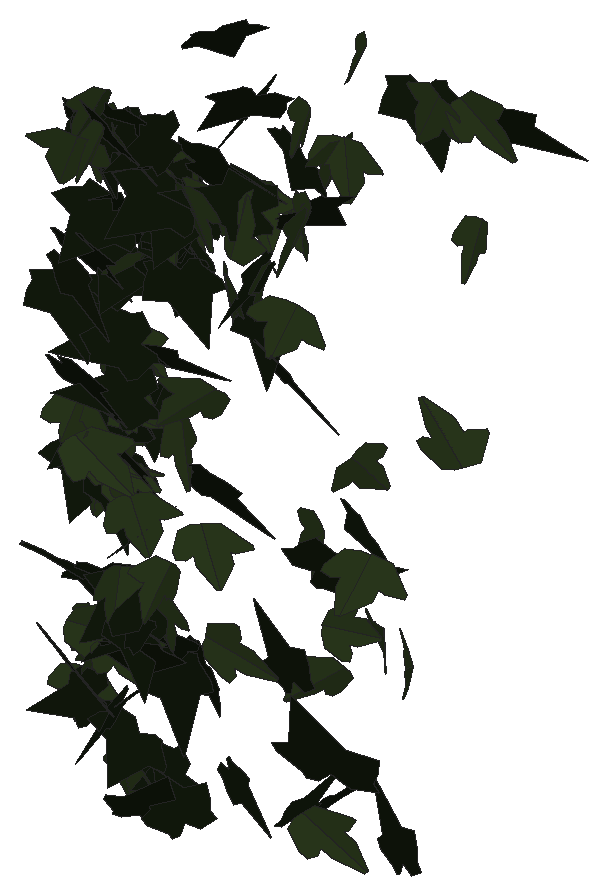
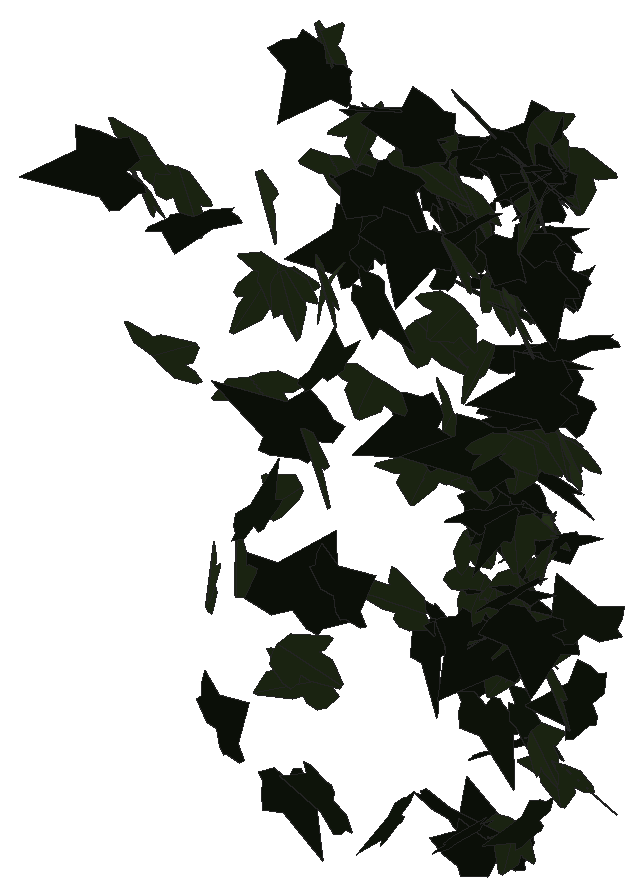
# SketchUp Ruby script. Lengths in inches.
U = 1.inch
M = Sketchup.active_model
def pt(a) = Geom::Point3d.new(a.map { |v| v * U })
def face(e, loops, mat)
  f = e.add_face(loops[0].map { |a| pt(a) })
  loops[1..].each { |l| e.add_face(l.map { |a| pt(a) }).erase! }
  f.material = f.back_material = mat if mat
  f
end
# faces: each face lists its corners as indices into pts; further lists are holes
def faces(e, pts, list, mat = nil) = list.each { |f| face(e, (f[0].is_a?(Array) ? f : [f]).map { |l| l.map { |i| pts[i] } }, mat) }
# xy, xz, yz: faces in a plane at the given z, y or x. An outline is a flat list of corners, or four numbers for a rectangle; further outlines are holes
def ring(l) = l.size == 4 ? [[l[0], l[1]], [l[2], l[1]], [l[2], l[3]], [l[0], l[3]]] : l.each_slice(2).to_a
def flat(e, list, mat, &to3) = list.each { |f| face(e, (f[0].is_a?(Array) ? f : [f]).map { |l| ring(l).map { |u, v| to3.(u, v) } }, mat) }
def xy(e, z, list, mat = nil) = flat(e, list, mat) { |x, y| [x, y, z] }
def xz(e, y, list, mat = nil) = flat(e, list, mat) { |x, z| [x, y, z] }
def yz(e, x, list, mat = nil) = flat(e, list, mat) { |y, z| [x, y, z] }
def lines(e, pts, list) = list.each { |a, b| e.add_line(pt(pts[a]), pt(pts[b])) }
# prism: a flat outline (further loops are holes) pulled along v
def prism(e, loops, v, mat = nil)
  f = face(e, loops, mat); d = Geom::Vector3d.new(v.map { |x| x * U })
  f.pushpull(f.normal.samedirection?(d) ? d.length : -d.length)
end
def box(e, o, s, mat = nil) = prism(e, [[o, [o[0] + s[0], o[1], o[2]], [o[0] + s[0], o[1] + s[1], o[2]], [o[0], o[1] + s[1], o[2]]]], [0, 0, s[2]], mat)
def at(x, y, z, deg = 0) = Geom::Transformation.translation(pt([x, y, z])) * Geom::Transformation.rotation(ORIGIN, Z_AXIS, deg.degrees)
def axes(o, x, y, z) = Geom::Transformation.new([*x, 0, *y, 0, *z, 0, *pt(o).to_a, 1])
def part(name) = M.definitions.add(name)
# library, detail: a bought-in or finely detailed component or shape, given as its bounding box
def library(name, o, s) = part(name).tap { |d| box(d.entities, o, s) }
def detail(e, o, s) = box(e.add_group.entities, o, s)
def put(e, d, t, mat = nil) = e.add_instance(d, t).tap { |i| i.material = mat if mat }
def group(e, t, mat = nil) = e.add_group.tap { |g| g.transformation = t; g.material = mat if mat }.entities
root = M.entities
M.materials.add("1026 AP 7946 SUNNY SIDE UP").color = [254, 231, 186]
M.materials.add("efeu1").color = [18, 25, 13]
M.materials.add("efeu2").color = [43, 57, 29]
c1 = part("ivyleaf_9")
p = [[1.54,2.16,1.25],[1.36,2.04,1.19],[-0.21,0.99,0.68],[-0.71,1.11,0.82],[-0.85,0.86,0.67],[-0.8,0.17,0.21],
  [-0.9,-0.01,0.1],[-0.67,-0.16,-0.02],[-0.08,-0.08,-0.05],[-0.03,-0.6,-0.4],[0.65,-0.88,-0.66],[0.83,-0.6,-0.49],
  [1.29,-0.42,-0.43],[1.8125,-0.07,-0.26],[1.21,0.44,0.15]]
faces(c1.entities,p,[[0,1,2,3,4,5,6,7,8,9,10,11,12,13,14]],"efeu1")
c2 = part("ivyleaf_10")
p = [[0,0.5,-0.03],[-0.0625,2.02,-0.43],[-0.19,2.01,-0.46],[-0.54,1.05,-0.29],[-0.52,0.625,-0.18],[-0.83,0.76,-0.28],
  [-1.16,0.64,-0.33],[-1.15,0.33,-0.24],[-0.77,-0.39,0.02],[-0.3,-0.51,0.16],[0.04,-0.48,0.23],[-0.02,2.01,-0.4375],
  [-0.06,2.01,-0.43],[0.04,-0.49,0.23],[0.67,-0.49,0.14],[1.38,0.36,-0.2],[1.375,0.51,-0.24],[0.81,0.65,-0.19],
  [0.62,0.59,-0.15],[0.6,1.09,-0.28],[0.5,1.23,-0.31]]
faces(c2.entities,p,[[0,1,2,3,4,5,6,7,8,9,10],[11,12,0,13,14,15,16,17,18,19,20]],"efeu2")
put(root,c1,axes([146.78,212.04,288.875],[-0.23408,-0.17766,-0.27786],[0.44088,0.07427,-0.21018],[0.24937,-0.29808,0.11077]),"1026 AP 7946 SUNNY SIDE UP")
put(root,c1,axes([145.62,212.05,281.24],[-0.34085,0.15175,-0.24525],[0.25955,-0.17669,-0.27093],[-0.36154,-0.26991,0.03672]),"1026 AP 7946 SUNNY SIDE UP")
put(root,c2,axes([145.19,211.82,285.48],[0.2947,0.22643,0.2345],[0.28013,0.14416,-0.29969],[-0.41828,0.25608,-0.03549]),"1026 AP 7946 SUNNY SIDE UP")
put(root,c2,axes([146.36,212.14,283.64],[-0.13398,-0.26958,0.2337],[0.11728,-0.24336,-0.26869],[0.54303,-0.01395,0.11569]),"1026 AP 7946 SUNNY SIDE UP")
put(root,c2,axes([148.91,212.17,290.39],[0.14592,-0.29384,0.25942],[0.12371,-0.24098,-0.31886],[0.59753,0.12165,0.00266]),"1026 AP 7946 SUNNY SIDE UP")
put(root,c2,axes([145.15,212.07,290.55],[0.3062,-0.3038,0.05867],[0.01993,-0.06144,-0.37141],[0.48612,0.19388,-0.02173]),"1026 AP 7946 SUNNY SIDE UP")
put(root,c1,axes([145.82,212.17,282.5],[0.01041,-0.34577,0.06714],[0.00257,-0.06711,-0.35667],[0.55384,0.00681,0.00039]),"1026 AP 7946 SUNNY SIDE UP")
put(root,c1,axes([144.33,212.11,281.78],[0.39728,-0.24681,0.1217],[0.1027,-0.1037,-0.3634],[0.4188,0.25956,-0.02633]),"1026 AP 7946 SUNNY SIDE UP")
put(root,c1,axes([146.03,212.08,282.79],[-0.48631,0.1752,-0.10012],[0.10272,-0.08271,-0.36454],[-0.29862,-0.31377,0.03765]),"1026 AP 7946 SUNNY SIDE UP")
put(root,c1,axes([145.91,212.24,283.03],[-0.46982,-0.17159,0.08652],[-0.07672,-0.08404,-0.35211],[0.29113,-0.29905,0.04684]),"1026 AP 7946 SUNNY SIDE UP")
put(root,c2,axes([145.625,212.0625,283.32],[0.18037,0.34237,-0.09211],[-0.10693,-0.07297,-0.37011],[-0.54682,0.1272,0.04199]),"1026 AP 7946 SUNNY SIDE UP")
put(root,c1,axes([149.52,212.09,281.48],[0.47249,-0.0771,0.30815],[-0.42073,0.14472,0.31574],[-0.244,-0.39885,0.05227]),"1026 AP 7946 SUNNY SIDE UP")
put(root,c1,axes([146.42,212.25,289.92],[-0.48379,-0.14997,0.08644],[-0.0842,-0.08165,-0.34953],[0.25745,-0.30851,0.04813]),"1026 AP 7946 SUNNY SIDE UP")
put(root,c1,axes([146.6,212.21,282.15],[-0.37575,-0.06026,-0.35511],[0.54931,-0.0255,-0.2453],[0.02064,-0.41837,0.06358]),"1026 AP 7946 SUNNY SIDE UP")
put(root,c1,axes([145.75,212.3125,280.67],[-0.24404,-0.27844,0.14053],[-0.01992,-0.14845,-0.32413],[0.48823,-0.14523,0.05702]),"1026 AP 7946 SUNNY SIDE UP")
put(root,c1,axes([144.5625,212.15,288.18],[0.27699,-0.31072,-0.05424],[-0.05889,0.03722,-0.36747],[0.49158,0.17954,-0.01346]),"1026 AP 7946 SUNNY SIDE UP")
put(root,c2,axes([145.92,212.01,284.65],[0.35267,0.27992,0.09055],[0.02676,0.09606,-0.36598],[-0.45981,0.22029,0.04815]),"1026 AP 7946 SUNNY SIDE UP")
put(root,c1,axes([144.61,212.08,286.51],[0.5392,-0.07749,0.00335],[-0.00561,-0.03248,-0.36082],[0.12186,0.34139,-0.03145]),"1026 AP 7946 SUNNY SIDE UP")
put(root,c2,axes([145.08,211.89,282.43],[0.1246,0.10429,0.35766],[0.21837,0.31888,-0.12969],[-0.52556,0.15722,0.03091]),"1026 AP 7946 SUNNY SIDE UP")
put(root,c2,axes([144.69,212.2,285.77],[0.53061,-0.06171,0.06348],[0.08715,-0.04015,-0.35237],[0.10637,0.34074,-0.02794]),"1026 AP 7946 SUNNY SIDE UP")
put(root,c2,axes([148.69,212.1875,288.76],[0.55055,-0.00188,-0.0654],[-0.09982,-0.00395,-0.36071],[0.0018,0.35582,-0.00227]),"1026 AP 7946 SUNNY SIDE UP")
put(root,c2,axes([148.99,212.12,290.6],[0.22769,-0.32292,-0.12263],[-0.08393,0.10449,-0.36392],[0.5336,0.15423,-0.00491]),"1026 AP 7946 SUNNY SIDE UP")
put(root,c2,axes([144.6875,212.18,290.22],[-0.49181,-0.1449,0.09139],[-0.10414,-0.06901,-0.35383],[0.24675,-0.31794,0.03282]),"1026 AP 7946 SUNNY SIDE UP")
put(root,c1,axes([144.22,212.36,283.06],[-0.12655,-0.24153,0.19845],[0.3527,-0.18369,-0.1408],[0.33599,0.10185,0.22255]),"1026 AP 7946 SUNNY SIDE UP")
put(root,c2,axes([147.14,212.14,284.52],[0.39354,0.24512,0.07196],[0.09352,0.03702,-0.36035],[-0.38909,0.25682,-0.01384]),"1026 AP 7946 SUNNY SIDE UP")
put(root,c1,axes([145.85,212.02,282.23],[0.49638,0.18393,-0.04541],[-0.03763,-0.04827,-0.37545],[-0.29541,0.31521,-0.02848]),"1026 AP 7946 SUNNY SIDE UP")
put(root,c2,axes([146.97,212.33,286.77],[-0.27638,-0.20571,0.24816],[-0.22149,-0.19749,-0.27942],[0.4477,-0.22469,0.01496]),"1026 AP 7946 SUNNY SIDE UP")
put(root,c2,axes([149.2,212.13,280.43],[0.31899,0.07924,0.30103],[0.42366,0.11199,-0.22368],[-0.21563,0.33725,0.00585]),"1026 AP 7946 SUNNY SIDE UP")
put(root,c2,axes([144.57,212.16,285.44],[0.38101,-0.27928,0.07261],[-0.04558,0.07007,0.38054],[-0.45124,-0.24289,0.02287]),"1026 AP 7946 SUNNY SIDE UP")
put(root,c2,axes([146.8,212.26,290.02],[-0.42848,0.1815,-0.13425],[0.13124,-0.10969,-0.33518],[-0.32693,-0.28191,0.0414]),"1026 AP 7946 SUNNY SIDE UP")
put(root,c1,axes([146.07,212.18,284.31],[-0.19556,0.32748,-0.08723],[0.02994,-0.08527,-0.36116],[-0.53176,-0.12523,0.01174]),"1026 AP 7946 SUNNY SIDE UP")
put(root,c2,axes([149.97,212.35,284.93],[0.43847,0.21787,-0.15486],[-0.16523,-0.11123,-0.36457],[-0.38322,0.29725,-0.02]),"1026 AP 7946 SUNNY SIDE UP")
put(root,c1,axes([146.49,212.5,289.78],[-0.32208,-0.3125,0.04839],[-0.01557,-0.05171,-0.38468],[0.49707,-0.2041,0.01931]),"1026 AP 7946 SUNNY SIDE UP")
put(root,c2,axes([145.53,212.125,282.16],[0.33896,0.23804,0.18488],[0.07945,0.18747,-0.32002],[-0.46068,0.20748,0.08084]),"1026 AP 7946 SUNNY SIDE UP")
put(root,c1,axes([148.1,212.41,288.5],[-0.36024,-0.04808,-0.29016],[0.44816,-0.0183,-0.23595],[0.02516,-0.3624,0.04825]),"1026 AP 7946 SUNNY SIDE UP")
put(root,c1,axes([145.03,212.55,289.06],[-0.35761,-0.25109,0.1144],[-0.09275,-0.09804,-0.34891],[0.42256,-0.23401,0.02024]),"1026 AP 7946 SUNNY SIDE UP")
put(root,c1,axes([144.59,212.25,288.55],[0.53791,-0.05822,-0.01309],[-0.02757,-0.02956,-0.35614],[0.08944,0.34104,-0.03104]),"1026 AP 7946 SUNNY SIDE UP")
put(root,c2,axes([146.15,212.28,283.0625],[-0.49724,0.17178,-0.0386],[0.03365,-0.04093,-0.37004],[-0.27473,-0.31592,0.02453]),"1026 AP 7946 SUNNY SIDE UP")
put(root,c2,axes([147.66,212.25,289.53],[0.45942,-0.20485,0.07516],[-0.06763,0.06732,0.36672],[-0.3358,-0.29382,0.02898]),"1026 AP 7946 SUNNY SIDE UP")
put(root,c1,axes([144.34,212.45,287.61],[-0.12644,-0.32611,-0.11379],[0.10828,0.09399,-0.34272],[0.5295,-0.09709,0.04291]),"1026 AP 7946 SUNNY SIDE UP")
put(root,c1,axes([148.11,212.4,287.75],[0.48822,-0.2183,0.09883],[0.09779,-0.08002,-0.39036],[0.36277,0.31535,-0.02778]),"1026 AP 7946 SUNNY SIDE UP")
put(root,c1,axes([147.93,212.53,289.13],[-0.37813,0.10771,-0.24609],[0.27352,-0.17793,-0.26343],[-0.30932,-0.28901,0.0679]),"1026 AP 7946 SUNNY SIDE UP")
put(root,c1,axes([145.52,212.59,287.01],[-0.39329,-0.08168,0.24096],[-0.32174,-0.12044,-0.26892],[0.22086,-0.3209,0.03734]),"1026 AP 7946 SUNNY SIDE UP")
put(root,c1,axes([146.7,212.28,288.71],[-0.08226,-0.02513,-0.37414],[-0.57199,-0.00644,0.05442],[-0.01568,0.36673,-0.02252]),"1026 AP 7946 SUNNY SIDE UP")
put(root,c1,axes([144.78,212.47,290.55],[0.39045,-0.20251,0.16043],[0.15525,-0.12594,-0.32922],[0.37167,0.26535,-0.03101]),"1026 AP 7946 SUNNY SIDE UP")
put(root,c1,axes([144.86,212.41,280.96],[-0.43576,0.16682,0.05124],[-0.08855,0.00068,-0.33196],[-0.25855,-0.28139,0.02734]),"1026 AP 7946 SUNNY SIDE UP")
put(root,c2,axes([144.8,212.38,282.16],[0.28114,-0.2518,-0.12915],[-0.11498,0.10007,-0.31756],[0.42604,0.19317,-0.00048]),"1026 AP 7946 SUNNY SIDE UP")
put(root,c1,axes([146.86,212.37,285.33],[0.55125,-0.0633,0.07074],[0.09762,-0.04319,-0.36588],[0.11026,0.35469,-0.02975]),"1026 AP 7946 SUNNY SIDE UP")
put(root,c2,axes([146.3125,212.58,285.8],[0.37335,-0.1573,0.26624],[0.3434,-0.13987,-0.29422],[0.33095,0.32259,0.00494]),"1026 AP 7946 SUNNY SIDE UP")
put(root,c2,axes([144.76,212.59,290.82],[-0.0327,-0.30541,0.18331],[0.02719,-0.18064,-0.31533],[0.5565,-0.00912,0.02618]),"1026 AP 7946 SUNNY SIDE UP")
put(root,c1,axes([145.55,212.63,286.1],[-0.3321,-0.04107,0.28153],[-0.37936,-0.14092,-0.21455],[0.21265,-0.31553,0.05693]),"1026 AP 7946 SUNNY SIDE UP")
put(root,c1,axes([144.95,212.54,285.44],[-0.51709,-0.00132,-0.0316],[0.04825,-0.02193,-0.33816],[-0.00114,-0.32955,0.02069]),"1026 AP 7946 SUNNY SIDE UP")
put(root,c1,axes([146.17,212.48,290.6875],[-0.48846,0.16461,-0.0372],[0.02853,-0.04457,-0.36105],[-0.26377,-0.30965,0.02983]),"1026 AP 7946 SUNNY SIDE UP")
put(root,c2,axes([146.1,212.59,289.4],[0.38334,-0.13282,0.23633],[0.29815,-0.13187,-0.28609],[0.29273,0.30825,-0.01809]),"1026 AP 7946 SUNNY SIDE UP")
put(root,c2,axes([147.89,212.58,289.03],[0.15648,-0.33005,0.08413],[0.10802,-0.06578,-0.35241],[0.52432,0.11205,0.0475]),"1026 AP 7946 SUNNY SIDE UP")
put(root,c1,axes([149,212.46,284.47],[0.08803,-0.03724,0.37168],[0.55489,-0.07968,-0.06531],[0.13321,0.35652,0.02644]),"1026 AP 7946 SUNNY SIDE UP")
put(root,c1,axes([147.74,212.61,289.99],[-0.37738,0.0624,0.26572],[-0.41672,-0.05852,-0.24013],[0.00242,-0.34716,0.08609]),"1026 AP 7946 SUNNY SIDE UP")
put(root,c1,axes([144.91,212.67,284.43],[0.09735,-0.33047,0.05524],[0.00051,-0.05638,-0.34655],[0.52692,0.06111,-0.00987]),"1026 AP 7946 SUNNY SIDE UP")
put(root,c2,axes([144.89,212.55,284.625],[-0.49152,0.09201,0.03179],[-0.09076,-0.09458,-0.31778],[-0.12234,-0.29948,0.10803]),"1026 AP 7946 SUNNY SIDE UP")
put(root,c1,axes([145.89,212.38,282.33],[0.48255,0.16934,-0.0123],[0.00064,-0.02737,-0.36039],[-0.26704,0.30594,-0.02308]),"1026 AP 7946 SUNNY SIDE UP")
put(root,c2,axes([147.08,212.55,282.51],[0.0697,0.01732,0.36866],[0.55916,0.04101,-0.04719],[-0.06739,0.35816,-0.0103]),"1026 AP 7946 SUNNY SIDE UP")
put(root,c2,axes([149.76,212.43,286.58],[-0.1707,-0.26951,-0.23903],[0.20086,0.19516,-0.29592],[0.5202,-0.16379,0.03582]),"1026 AP 7946 SUNNY SIDE UP")
put(root,c1,axes([145.32,212.76,288.4],[-0.38906,-0.24468,-0.00627],[0.02318,-0.00823,-0.35815],[0.38411,-0.24734,0.01526]),"1026 AP 7946 SUNNY SIDE UP")
put(root,c1,axes([146.89,212.46,282.16],[0.2365,-0.04799,-0.35181],[-0.52577,0.06962,-0.16152],[0.13091,0.36634,-0.01313]),"1026 AP 7946 SUNNY SIDE UP")
put(root,c1,axes([145.57,212.64,279.14],[0.50251,0.12568,0.09947],[-0.15946,-0.00278,0.35209],[0.19063,-0.33363,0.03231]),"1026 AP 7946 SUNNY SIDE UP")
put(root,c2,axes([147.29,212.53,288.65],[-0.32924,0.27881,0.06645],[-0.11445,0.02341,-0.35627],[-0.4346,-0.21738,0.04349]),"1026 AP 7946 SUNNY SIDE UP")
put(root,c1,axes([146.11,212.79,288.82],[-0.04952,-0.34903,0.0177],[0.04565,-0.02179,-0.35976],[0.54775,-0.02974,0.03158]),"1026 AP 7946 SUNNY SIDE UP")
put(root,c2,axes([145.15,212.65,284.71],[0.38331,0.21374,-0.05895],[-0.04423,-0.05632,-0.33345],[-0.3456,0.24427,-0.0227]),"1026 AP 7946 SUNNY SIDE UP")
put(root,c2,axes([145.2,212.58,290.24],[-0.33228,0.28203,-0.01745],[-0.00656,-0.02625,-0.36268],[-0.44438,-0.2105,0.0184]),"1026 AP 7946 SUNNY SIDE UP")
put(root,c1,axes([146.36,212.72,289.04],[-0.35175,0.15277,-0.2329],[0.27302,-0.14726,-0.2793],[-0.33243,-0.28259,0.01705]),"1026 AP 7946 SUNNY SIDE UP")
put(root,c1,axes([146.4375,212.51,279.4],[0.02805,0.154,0.31348],[-0.37148,0.22427,-0.10164],[-0.38505,-0.20515,0.1209]),"1026 AP 7946 SUNNY SIDE UP")
put(root,c1,axes([144.9,212.5625,283.01],[0.30721,0.24351,-0.12077],[-0.08527,-0.10813,-0.32133],[-0.41728,0.20137,-0.02325]),"1026 AP 7946 SUNNY SIDE UP")
put(root,c1,axes([148.74,212.42,290.42],[0.27422,0.28873,0.12742],[0.12508,0.09433,-0.34644],[-0.47676,0.19082,-0.0176]),"1026 AP 7946 SUNNY SIDE UP")
put(root,c2,axes([144.41,212.71,280.97],[0.4948,0.03068,0.01723],[0.02698,-0.00545,-0.32566],[-0.04771,0.31506,-0.00544]),"1026 AP 7946 SUNNY SIDE UP")
put(root,c1,axes([144.48,212.88,284.61],[-0.2875,-0.29109,0.01857],[0.00591,-0.02557,-0.35386],[0.45872,-0.18211,0.0162]),"1026 AP 7946 SUNNY SIDE UP")
put(root,c1,axes([145.98,212.97,288.65],[-0.42638,-0.14348,0.16857],[0.16157,-0.31533,-0.11073],[0.30275,-0.0338,0.2965]),"1026 AP 7946 SUNNY SIDE UP")
put(root,c2,axes([145.4,212.75,288.3],[-0.11285,-0.34152,0.03316],[-0.00221,-0.03457,-0.35967],[0.53967,-0.07156,0.00546]),"1026 AP 7946 SUNNY SIDE UP")
put(root,c2,axes([146.9375,212.77,289.68],[-0.27684,-0.0559,0.30978],[-0.41833,-0.14391,-0.18868],[0.23824,-0.31765,0.02867]),"1026 AP 7946 SUNNY SIDE UP")
put(root,c1,axes([145.74,212.58,281.4],[-0.09036,0.34102,-0.02067],[0.00307,-0.02198,-0.35639],[-0.53732,-0.05747,0.00144]),"1026 AP 7946 SUNNY SIDE UP")
put(root,c1,axes([144.36,212.82,290.05],[0.31443,-0.1147,0.27724],[0.3257,-0.17578,-0.2362],[0.32614,0.28611,-0.0314]),"1026 AP 7946 SUNNY SIDE UP")
put(root,c2,axes([145.17,212.8,285.91],[0.54223,-0.04509,-0.00573],[-0.01435,-0.02905,-0.35711],[0.06993,0.34365,-0.02888]),"1026 AP 7946 SUNNY SIDE UP")
put(root,c1,axes([144.93,212.74,287.92],[0.31053,-0.2631,-0.09325],[0.41171,0.2128,-0.04827],[0.14575,-0.04055,0.33503]),"1026 AP 7946 SUNNY SIDE UP")
put(root,c1,axes([145.04,212.57,290.1],[-0.06756,0.20745,0.29157],[-0.31162,0.21962,-0.19637],[-0.45354,-0.18179,0.09149]),"1026 AP 7946 SUNNY SIDE UP")
put(root,c1,axes([144.95,212.71,285.05],[0.52531,-0.09766,-0.06462],[-0.10225,-0.00122,-0.35804],[0.15061,0.33981,-0.01771]),"1026 AP 7946 SUNNY SIDE UP")
put(root,c1,axes([144.44,212.95,290.11],[0.1132,-0.33567,0.06601],[0.01123,-0.06594,-0.35399],[0.5378,0.07203,-0.0065]),"1026 AP 7946 SUNNY SIDE UP")
put(root,c2,axes([145.18,212.75,279.73],[-0.45849,0.12766,-0.00742],[-0.00631,-0.02885,-0.32681],[-0.20101,-0.29026,0.02717]),"1026 AP 7946 SUNNY SIDE UP")
put(root,c1,axes([145.03,212.85,289.1],[-0.07303,0.22567,-0.26923],[-0.05921,-0.26669,-0.23079],[-0.54123,-0.00127,0.06158]),"1026 AP 7946 SUNNY SIDE UP")
put(root,c2,axes([144.98,212.67,285.68],[0.3368,-0.24892,0.0443],[0.39758,0.21062,-0.03893],[0.00166,0.05909,0.33626]),"1026 AP 7946 SUNNY SIDE UP")
put(root,c2,axes([147.67,212.74,290.04],[0.17905,0.3353,0.05073],[-0.00055,0.05006,-0.36412],[-0.53245,0.1127,0.01744]),"1026 AP 7946 SUNNY SIDE UP")
put(root,c2,axes([144.83,212.68,284.75],[0.33273,-0.24982,-0.00241],[0.39279,0.21161,-0.0014],[0.00401,0.00096,0.33727]),"1026 AP 7946 SUNNY SIDE UP")
put(root,c1,axes([148.3125,212.7,282.35],[0.10009,-0.07689,0.36088],[-0.23803,0.31726,0.10181],[-0.51198,-0.16253,0.02322]),"1026 AP 7946 SUNNY SIDE UP")
put(root,c1,axes([144.63,212.96,290.23],[-0.08361,-0.34247,-0.04916],[-0.00101,0.04641,-0.35668],[0.54329,-0.05262,-0.00823]),"1026 AP 7946 SUNNY SIDE UP")
put(root,c1,axes([146.47,212.85,290.25],[0.34082,-0.07867,0.27598],[0.37543,-0.12466,-0.23707],[0.22888,0.32163,-0.0221]),"1026 AP 7946 SUNNY SIDE UP")
put(root,c2,axes([149.26,212.57,283.55],[-0.0069,0.15063,0.34302],[0.0239,0.33192,-0.15294],[-0.57291,0.01203,-0.01051]),"1026 AP 7946 SUNNY SIDE UP")
put(root,c2,axes([144.53,212.95,281.45],[0.03894,-0.31546,0.09401],[0.021,-0.09227,-0.32647],[0.51673,0.02752,0.00618]),"1026 AP 7946 SUNNY SIDE UP")
put(root,c2,axes([145.75,212.92,289.64],[0.44764,-0.19951,-0.02879],[-0.0402,0.01024,-0.35801],[0.31397,0.28576,-0.00478]),"1026 AP 7946 SUNNY SIDE UP")
put(root,c1,axes([144.83,212.94,290.38],[-0.28395,-0.21209,-0.2201],[0.23721,0.15023,-0.28573],[0.40809,-0.23489,0.01294]),"1026 AP 7946 SUNNY SIDE UP")
put(root,c1,axes([144.33,212.83,286.97],[0.50717,-0.05082,0.14297],[0.21216,-0.03638,-0.3363],[0.09587,0.34936,-0.01212]),"1026 AP 7946 SUNNY SIDE UP")
put(root,c2,axes([144.42,212.91,284.51],[-0.04862,0.33441,-0.07671],[-0.00019,-0.07668,-0.34635],[-0.53937,-0.03012,0.00704]),"1026 AP 7946 SUNNY SIDE UP")
put(root,c1,axes([144.9,212.82,290.5625],[0.41042,0.07919,-0.23517],[-0.33845,-0.07794,-0.2813],[-0.1741,0.33819,-0.00757]),"1026 AP 7946 SUNNY SIDE UP")
put(root,c2,axes([144.76,212.93,290.28],[0.23411,-0.30219,-0.09183],[-0.08471,0.07079,-0.34622],[0.48734,0.15747,-0.01607]),"1026 AP 7946 SUNNY SIDE UP")
put(root,c1,axes([144.63,212.92,288.82],[0.33587,0.09159,-0.26385],[-0.34912,-0.13053,-0.23914],[-0.24838,0.30733,-0.02065]),"1026 AP 7946 SUNNY SIDE UP")
put(root,c2,axes([148.57,212.93,284.72],[0.29446,-0.26615,-0.21915],[-0.15795,0.18702,-0.33344],[0.51039,0.21143,0.02325]),"1026 AP 7946 SUNNY SIDE UP")
put(root,c1,axes([145.82,213.28,279.59],[-0.2158,-0.12403,0.2618],[-0.18339,-0.23334,-0.18307],[0.40616,-0.17125,0.05644]),"1026 AP 7946 SUNNY SIDE UP")
put(root,c1,axes([144.8,213.01,285.26],[-0.21924,0.16049,0.2599],[0.29643,-0.16759,0.21697],[0.36337,0.23354,-0.02019]),"1026 AP 7946 SUNNY SIDE UP")
put(root,c2,axes([144.63,212.84,289.84],[-0.01227,0.25022,0.25481],[-0.13762,0.23682,-0.2497],[-0.53422,-0.06675,0.05848]),"1026 AP 7946 SUNNY SIDE UP")
put(root,c1,axes([144.41,213.15,280.35],[0.32649,-0.23197,-0.04241],[-0.00969,0.04776,-0.31924],[0.36997,0.20596,0.02906]),"1026 AP 7946 SUNNY SIDE UP")
put(root,c2,axes([144.75,213.25,288.34],[0.31875,-0.27772,-0.00137],[-0.02824,-0.01341,-0.35354],[0.43578,0.20227,-0.02191]),"1026 AP 7946 SUNNY SIDE UP")
put(root,c1,axes([150.09,213.05,279.79],[0.11448,-0.1062,0.38223],[-0.16556,0.35842,0.12886],[-0.58477,-0.12226,0.03835]),"1026 AP 7946 SUNNY SIDE UP")
put(root,c1,axes([145.58,213.45,288.76],[0.08558,-0.22339,0.26692],[0.11538,-0.24994,-0.23818],[0.52694,0.09101,0.0088]),"1026 AP 7946 SUNNY SIDE UP")
put(root,c2,axes([144.74,213.24,284.9375],[-0.30587,-0.26332,0.00543],[0.02208,-0.01877,-0.33658],[0.41359,-0.19373,0.02199]),"1026 AP 7946 SUNNY SIDE UP")
put(root,c2,axes([144.6,213.26,286.21],[-0.5176,-0.0511,-0.01301],[0.02712,-0.03103,-0.34164],[0.07808,-0.32794,0.03238]),"1026 AP 7946 SUNNY SIDE UP")
put(root,c1,axes([145.41,213.59,289.5],[-0.0623,-0.34254,0.02832],[-0.00597,-0.02919,-0.3554],[0.54056,-0.0398,-0.00066]),"1026 AP 7946 SUNNY SIDE UP")
put(root,c1,axes([146.58,213.46,279.81],[0.29775,-0.23828,-0.10122],[-0.10567,0.07032,-0.31302],[0.39042,0.20075,-0.00752]),"1026 AP 7946 SUNNY SIDE UP")
put(root,c1,axes([146.78,213.75,288.7],[-0.09303,-0.10967,0.33704],[0.11535,-0.32896,-0.10166],[0.53111,0.05224,0.08112]),"1026 AP 7946 SUNNY SIDE UP")
put(root,c1,axes([144.45,213.67,284.16],[-0.02089,-0.32303,0.00025],[0.01022,-0.00234,-0.33301],[0.50785,-0.01324,0.00671]),"1026 AP 7946 SUNNY SIDE UP")
put(root,c1,axes([147.85,213.37,279.57],[-0.18529,0.30711,-0.06557],[-0.02036,0.06503,0.33906],[0.49331,0.11804,-0.01063]),"1026 AP 7946 SUNNY SIDE UP")
put(root,c2,axes([148.21,213.77,281.92],[-0.17134,-0.18715,0.27035],[-0.17995,-0.2377,-0.22408],[0.47525,-0.15748,0.01262]),"1026 AP 7946 SUNNY SIDE UP")
put(root,c2,axes([144.63,213.54,286.33],[-0.29702,-0.21644,-0.17753],[0.27057,0.06966,-0.28609],[0.33911,-0.24516,0.07277]),"1026 AP 7946 SUNNY SIDE UP")
put(root,c2,axes([149.17,213.72,282.6875],[-0.33191,0.21321,0.20638],[0.24486,-0.12549,0.30775],[0.38791,0.26164,-0.01767]),"1026 AP 7946 SUNNY SIDE UP")
put(root,c2,axes([149.55,213.87,282.4375],[-0.1733,0.1645,0.32996],[0.31753,-0.2479,0.20189],[0.46716,0.22952,-0.01482]),"1026 AP 7946 SUNNY SIDE UP")
put(root,c1,axes([144.74,213.8125,285.4],[-0.15708,-0.30636,-0.06737],[0.07904,0.05024,-0.33007],[0.48562,-0.10727,0.03193]),"1026 AP 7946 SUNNY SIDE UP")
put(root,c1,axes([144.78,213.61,286.16],[0.43253,-0.02389,0.19024],[0.29285,0.04585,-0.27921],[-0.00943,0.3282,0.05483]),"1026 AP 7946 SUNNY SIDE UP")
put(root,c1,axes([144.57,213.625,285.34],[0.3755,-0.08796,-0.21399],[-0.2867,0.10159,-0.26031],[0.20759,0.29941,0.02756]),"1026 AP 7946 SUNNY SIDE UP")
put(root,c2,axes([144.95,213.64,287.71],[-0.01988,0.26637,0.21863],[-0.09809,0.20544,-0.27021],[-0.52495,-0.04848,0.04221]),"1026 AP 7946 SUNNY SIDE UP")
put(root,c1,axes([148.26,213.78,279.88],[-0.09083,0.31868,-0.09151],[0.01111,-0.0908,-0.33405],[-0.52084,-0.05751,0.00883]),"1026 AP 7946 SUNNY SIDE UP")
put(root,c2,axes([145.32,213.92,289.41],[0.44192,-0.20236,0.00441],[-0.01588,-0.02329,-0.35599],[0.3179,0.28013,-0.02391]),"1026 AP 7946 SUNNY SIDE UP")
put(root,c2,axes([145.14,214.06,288.49],[-0.45952,0.08975,-0.15514],[0.18773,-0.11377,-0.30816],[-0.20279,-0.30869,0.06627]),"1026 AP 7946 SUNNY SIDE UP")
put(root,c1,axes([148.46,214.28,284.12],[0.30946,-0.2565,-0.12663],[0.14208,-0.08349,0.33197],[-0.42304,-0.21568,0.01886]),"1026 AP 7946 SUNNY SIDE UP")
put(root,c2,axes([150.19,214.19,286.11],[0.45653,0.05795,0.24089],[-0.3762,0.03109,0.2987],[0.03975,-0.37128,0.06037]),"1026 AP 7946 SUNNY SIDE UP")
put(root,c1,axes([146.125,214.5625,290.47],[-0.00486,0.23558,-0.26781],[-0.13229,-0.25422,-0.23658],[-0.53714,0.06048,0.06069]),"1026 AP 7946 SUNNY SIDE UP")
put(root,c2,axes([147.02,214.5,288.41],[0.00642,0.20692,-0.28985],[-0.10463,0.27786,0.21028],[0.54062,0.05132,0.04414]),"1026 AP 7946 SUNNY SIDE UP")
put(root,c2,axes([149.89,215.02,289.35],[0.40698,-0.2266,0.13679],[0.12654,-0.11092,-0.35383],[0.39419,0.26956,-0.02764]),"1026 AP 7946 SUNNY SIDE UP")
put(root,c2,axes([145.24,215.71,288.06],[0.52208,0.01183,0.1309],[0.19805,0.0254,-0.34153],[-0.03161,0.35457,0.02219]),"1026 AP 7946 SUNNY SIDE UP")
put(root,c2,axes([146.82,215.77,289.29],[0.5511,-0.0156,0.08506],[0.1309,0.01354,-0.36093],[0.01896,0.35984,0.01938]),"1026 AP 7946 SUNNY SIDE UP")
put(root,c1,axes([144.61,215.58,290.57],[0.23668,0.31614,0.0075],[0.01838,0.0005,-0.36056],[-0.49684,0.15062,-0.00977]),"1026 AP 7946 SUNNY SIDE UP")
put(root,c1,axes([145.23,215.89,289.62],[-0.3173,0.19894,-0.22997],[0.21187,-0.18143,-0.29165],[-0.42121,-0.24113,0.02654]),"1026 AP 7946 SUNNY SIDE UP")
put(root,c2,axes([146.01,215.84,289.55],[0.31598,-0.28413,-0.0109],[0.01799,0.01906,-0.35779],[0.44663,0.20025,0.02212]),"1026 AP 7946 SUNNY SIDE UP")
put(root,c2,axes([146.61,215.91,289.21],[-0.04651,-0.35881,0.01993],[0.01366,-0.02216,-0.37087],[0.56503,-0.029,0.01061]),"1026 AP 7946 SUNNY SIDE UP")
put(root,c2,axes([148.92,216.1,290.54],[0.32586,0.00585,0.31135],[0.47378,0.02493,-0.21322],[-0.03752,0.36558,0.01171]),"1026 AP 7946 SUNNY SIDE UP")
put(root,c1,axes([145.54,216.43,288.42],[-0.13019,-0.20242,0.28995],[0.04801,-0.29362,-0.20916],[0.54448,-0.02251,0.08777]),"1026 AP 7946 SUNNY SIDE UP")
put(root,c2,axes([146.84,216.13,290.79],[0.15726,-0.32105,-0.10996],[-0.05822,0.09834,-0.34579],[0.52789,0.10649,-0.00538]),"1026 AP 7946 SUNNY SIDE UP")
put(root,c2,axes([148.28,216.16,290.38],[-0.49289,0.13736,0.13612],[-0.25104,-0.05287,-0.33586],[-0.16213,-0.33573,0.10624]),"1026 AP 7946 SUNNY SIDE UP")
put(root,c1,axes([149.14,216.35,290.33],[0.46658,0.03935,0.21761],[0.33522,-0.01223,-0.30658],[-0.03919,0.3639,-0.03168]),"1026 AP 7946 SUNNY SIDE UP")
put(root,c1,axes([147.68,216.59,290.21],[-0.12308,-0.33331,-0.12946],[0.05824,0.1184,-0.35191],[0.55602,-0.08618,0.0082]),"1026 AP 7946 SUNNY SIDE UP")
